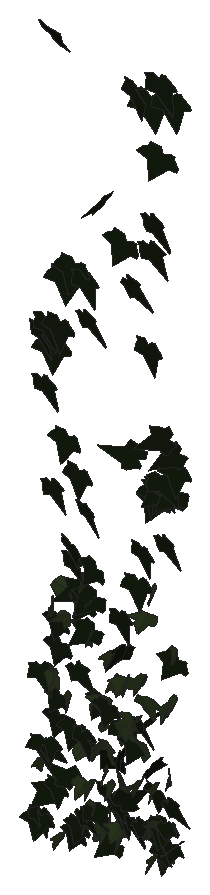
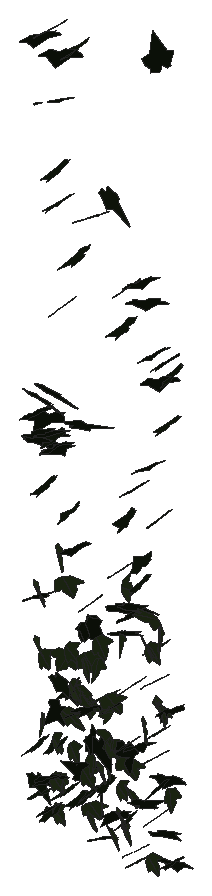
# SketchUp Ruby script. Lengths in inches.
U = 1.inch
M = Sketchup.active_model
def pt(a) = Geom::Point3d.new(a.map { |v| v * U })
def face(e, loops, mat)
  f = e.add_face(loops[0].map { |a| pt(a) })
  loops[1..].each { |l| e.add_face(l.map { |a| pt(a) }).erase! }
  f.material = f.back_material = mat if mat
  f
end
# faces: each face lists its corners as indices into pts; further lists are holes
def faces(e, pts, list, mat = nil) = list.each { |f| face(e, (f[0].is_a?(Array) ? f : [f]).map { |l| l.map { |i| pts[i] } }, mat) }
# xy, xz, yz: faces in a plane at the given z, y or x. An outline is a flat list of corners, or four numbers for a rectangle; further outlines are holes
def ring(l) = l.size == 4 ? [[l[0], l[1]], [l[2], l[1]], [l[2], l[3]], [l[0], l[3]]] : l.each_slice(2).to_a
def flat(e, list, mat, &to3) = list.each { |f| face(e, (f[0].is_a?(Array) ? f : [f]).map { |l| ring(l).map { |u, v| to3.(u, v) } }, mat) }
def xy(e, z, list, mat = nil) = flat(e, list, mat) { |x, y| [x, y, z] }
def xz(e, y, list, mat = nil) = flat(e, list, mat) { |x, z| [x, y, z] }
def yz(e, x, list, mat = nil) = flat(e, list, mat) { |y, z| [x, y, z] }
def lines(e, pts, list) = list.each { |a, b| e.add_line(pt(pts[a]), pt(pts[b])) }
# prism: a flat outline (further loops are holes) pulled along v
def prism(e, loops, v, mat = nil)
  f = face(e, loops, mat); d = Geom::Vector3d.new(v.map { |x| x * U })
  f.pushpull(f.normal.samedirection?(d) ? d.length : -d.length)
end
def box(e, o, s, mat = nil) = prism(e, [[o, [o[0] + s[0], o[1], o[2]], [o[0] + s[0], o[1] + s[1], o[2]], [o[0], o[1] + s[1], o[2]]]], [0, 0, s[2]], mat)
def at(x, y, z, deg = 0) = Geom::Transformation.translation(pt([x, y, z])) * Geom::Transformation.rotation(ORIGIN, Z_AXIS, deg.degrees)
def axes(o, x, y, z) = Geom::Transformation.new([*x, 0, *y, 0, *z, 0, *pt(o).to_a, 1])
def part(name) = M.definitions.add(name)
# library, detail: a bought-in or finely detailed component or shape, given as its bounding box
def library(name, o, s) = part(name).tap { |d| box(d.entities, o, s) }
def detail(e, o, s) = box(e.add_group.entities, o, s)
def put(e, d, t, mat = nil) = e.add_instance(d, t).tap { |i| i.material = mat if mat }
def group(e, t, mat = nil) = e.add_group.tap { |g| g.transformation = t; g.material = mat if mat }.entities
root = M.entities
M.materials.add("1026 AP 7946 SUNNY SIDE UP").color = [254, 231, 186]
M.materials.add("efeu1").color = [18, 25, 13]
M.materials.add("efeu2").color = [43, 57, 29]
c1 = part("ivyleaf_9")
p = [[1.54,2.16,1.25],[1.36,2.04,1.19],[-0.21,0.99,0.68],[-0.71,1.11,0.82],[-0.85,0.86,0.67],[-0.8,0.17,0.21],
  [-0.9,-0.01,0.1],[-0.67,-0.16,-0.02],[-0.08,-0.08,-0.05],[-0.03,-0.6,-0.4],[0.65,-0.88,-0.66],[0.83,-0.6,-0.49],
  [1.29,-0.42,-0.43],[1.8125,-0.07,-0.26],[1.21,0.44,0.15]]
faces(c1.entities,p,[[0,1,2,3,4,5,6,7,8,9,10,11,12,13,14]],"efeu1")
c2 = part("ivyleaf_10")
p = [[0,0.5,-0.03],[-0.0625,2.02,-0.43],[-0.19,2.01,-0.46],[-0.54,1.05,-0.29],[-0.52,0.625,-0.18],[-0.83,0.76,-0.28],
  [-1.16,0.64,-0.33],[-1.15,0.33,-0.24],[-0.77,-0.39,0.02],[-0.3,-0.51,0.16],[0.04,-0.48,0.23],[-0.02,2.01,-0.4375],
  [-0.06,2.01,-0.43],[0.04,-0.49,0.23],[0.67,-0.49,0.14],[1.38,0.36,-0.2],[1.375,0.51,-0.24],[0.81,0.65,-0.19],
  [0.62,0.59,-0.15],[0.6,1.09,-0.28],[0.5,1.23,-0.31]]
faces(c2.entities,p,[[0,1,2,3,4,5,6,7,8,9,10],[11,12,0,13,14,15,16,17,18,19,20]],"efeu2")
put(root,c1,axes([118.96,212.625,291.69],[0.00365,-0.3577,-0.01819],[0.01017,0.01567,-0.36835],[0.56289,0.00204,0.00677]),"1026 AP 7946 SUNNY SIDE UP")
put(root,c1,axes([119.125,212.41,291.59],[-0.41683,-0.22703,-0.10617],[0.19274,0.01023,-0.35238],[0.34043,-0.28377,0.06951]),"1026 AP 7946 SUNNY SIDE UP")
put(root,c1,axes([118.87,212.65,315.31],[0.20981,-0.41083,0.07483],[0.01065,-0.07657,-0.4451],[0.65657,0.13252,-0.01669]),"1026 AP 7946 SUNNY SIDE UP")
put(root,c1,axes([119.18,212.4,298.92],[-0.00879,-0.36906,-0.13016],[0.01023,0.12416,-0.3795],[0.61224,-0.00737,0.00447]),"1026 AP 7946 SUNNY SIDE UP")
put(root,c2,axes([119.4,212.16,294.67],[-0.0589,-0.36928,-0.07771],[0.03853,0.07115,-0.38157],[0.59074,-0.04146,0.01714]),"1026 AP 7946 SUNNY SIDE UP")
put(root,c1,axes([119.08,212.63,312.84],[0.20023,-0.41314,0.00123],[0.03723,0.0036,-0.44468],[0.64858,0.12734,0.02515]),"1026 AP 7946 SUNNY SIDE UP")
put(root,c1,axes([119.625,212.625,292.91],[-0.47533,-0.19178,0.08981],[-0.07174,-0.09117,-0.36558],[0.32412,-0.30143,0.05079]),"1026 AP 7946 SUNNY SIDE UP")
put(root,c1,axes([119.25,212.66,315.86],[0.07475,-0.4373,-0.03649],[-0.00062,0.03309,-0.45296],[0.68956,0.04743,0.00355]),"1026 AP 7946 SUNNY SIDE UP")
put(root,c1,axes([119.48,212.28,295.48],[-0.29395,-0.27444,-0.18053],[0.21651,0.11453,-0.33844],[0.46252,-0.22803,0.04369]),"1026 AP 7946 SUNNY SIDE UP")
put(root,c2,axes([119.64,212.49,298.83],[0.3553,-0.3055,-0.0603],[-0.00291,0.0689,-0.38899],[0.4886,0.22257,0.04153]),"1026 AP 7946 SUNNY SIDE UP")
put(root,c1,axes([119.57,212.32,295.24],[0.29152,-0.15965,-0.29131],[-0.19492,0.26508,-0.23712],[0.47059,0.20869,0.08224]),"1026 AP 7946 SUNNY SIDE UP")
put(root,c1,axes([119.67,212.66,314.85],[-0.26572,-0.39782,-0.07221],[0.05002,0.06018,-0.44489],[0.63259,-0.17186,0.00485]),"1026 AP 7946 SUNNY SIDE UP")
put(root,c1,axes([119.81,212.78,297.625],[-0.18055,-0.28615,0.22776],[-0.03288,-0.22799,-0.31422],[0.5692,-0.10393,0.05409]),"1026 AP 7946 SUNNY SIDE UP")
put(root,c1,axes([119.78,212.86,296.55],[-0.15027,-0.33014,0.15159],[0.00189,-0.15441,-0.35252],[0.56955,-0.08659,0.04116]),"1026 AP 7946 SUNNY SIDE UP")
put(root,c2,axes([119.92,212.2,302.37],[0.18565,-0.35673,-0.14226],[0.04747,0.1507,-0.37916],[0.59846,0.09871,0.0742]),"1026 AP 7946 SUNNY SIDE UP")
put(root,c2,axes([119.91,212.24,298.75],[0.51817,-0.19118,-0.02137],[-0.03149,0.00465,-0.39241],[0.30055,0.33009,-0.00427]),"1026 AP 7946 SUNNY SIDE UP")
put(root,c1,axes([119.68,212.4375,308.0625],[0.20165,-0.39278,-0.05654],[-0.01046,0.0532,-0.42522],[0.62304,0.12802,0.01116]),"1026 AP 7946 SUNNY SIDE UP")
put(root,c2,axes([120.03,212.25,298.87],[0.25373,-0.34513,-0.02903],[-0.04682,0.01498,-0.39184],[0.54224,0.16279,-0.02025]),"1026 AP 7946 SUNNY SIDE UP")
put(root,c1,axes([119.92,212.79,300.125],[-0.16934,-0.33464,0.16899],[-0.00213,-0.17235,-0.35997],[0.58733,-0.09711,0.04742]),"1026 AP 7946 SUNNY SIDE UP")
put(root,c1,axes([119.67,212.45,330.08],[0.64208,-0.18839,-0.15741],[0.24623,-0.02102,0.46093],[-0.28989,-0.43511,0.04286]),"1026 AP 7946 SUNNY SIDE UP")
put(root,c2,axes([120.14,212.61,301.58],[0.01087,-0.35287,0.17647],[0.00565,-0.17327,-0.36461],[0.61814,0.00779,0.00023]),"1026 AP 7946 SUNNY SIDE UP")
put(root,c1,axes([119.96,212.51,293.42],[-0.02179,-0.35642,0.10657],[-0.00696,-0.10538,-0.36808],[0.58442,-0.01455,-0.00041]),"1026 AP 7946 SUNNY SIDE UP")
put(root,c1,axes([119.97,212.66,315.95],[-0.09002,-0.43165,0.06713],[0.00279,-0.06842,-0.44884],[0.687,-0.05628,0.01062]),"1026 AP 7946 SUNNY SIDE UP")
put(root,c1,axes([120.07,212.45,301.55],[-0.14666,-0.32636,0.19998],[0.02445,-0.20487,-0.34505],[0.59808,-0.07165,0.06314]),"1026 AP 7946 SUNNY SIDE UP")
put(root,c2,axes([120.36,212.27,291.16],[-0.01751,-0.34657,0.10837],[-0.00014,-0.10721,-0.35783],[0.5704,-0.01067,0.00324]),"1026 AP 7946 SUNNY SIDE UP")
put(root,c1,axes([120.72,212.5,293.8125],[-0.08315,0.17554,0.32686],[-0.56814,-0.04091,-0.03908],[0.02719,-0.31806,0.18297]),"1026 AP 7946 SUNNY SIDE UP")
put(root,c2,axes([120.32,212.59,301.71],[0.47823,-0.22974,0.09619],[0.07621,-0.09191,-0.39072],[0.38321,0.30498,-0.04233]),"1026 AP 7946 SUNNY SIDE UP")
put(root,c1,axes([120.3,212.76,310.4],[-0.20744,-0.38508,0.1151],[0.01055,-0.122,-0.41758],[0.63136,-0.12448,0.04479]),"1026 AP 7946 SUNNY SIDE UP")
put(root,c2,axes([120,212.65,303.16],[-0.22612,-0.10451,-0.36375],[0.55616,-0.14264,-0.10592],[-0.1578,-0.35297,0.14792]),"1026 AP 7946 SUNNY SIDE UP")
put(root,c1,axes([120.34,212.74,318.45],[-0.33209,-0.38826,-0.07865],[0.14716,0.03256,-0.45007],[0.60386,-0.22145,0.06643]),"1026 AP 7946 SUNNY SIDE UP")
put(root,c2,axes([120.54,212.54,297.81],[0.2772,-0.33596,-0.06476],[0.01722,0.07413,-0.38784],[0.53661,0.17117,0.0459]),"1026 AP 7946 SUNNY SIDE UP")
put(root,c1,axes([120.71,212.86,291.18],[-0.17628,-0.29329,0.17103],[0.00192,-0.17703,-0.31917],[0.53122,-0.09669,0.05791]),"1026 AP 7946 SUNNY SIDE UP")
put(root,c1,axes([120.53,212.7,304.66],[0.24555,-0.37449,0.00065],[-0.01355,-0.00658,-0.41789],[0.5887,0.15605,-0.00989]),"1026 AP 7946 SUNNY SIDE UP")
put(root,c1,axes([120.8125,212.6,319.11],[-0.22944,-0.42315,0.05642],[0.00277,-0.06102,-0.46095],[0.67141,-0.14435,0.02119]),"1026 AP 7946 SUNNY SIDE UP")
put(root,c1,axes([120.89,212.86,291.62],[-0.16329,-0.3084,0.15046],[0.0019,-0.15479,-0.33278],[0.53774,-0.0931,0.04686]),"1026 AP 7946 SUNNY SIDE UP")
put(root,c1,axes([120.71,212.5,305.38],[0.07562,-0.32788,0.24609],[0.1049,-0.23278,-0.3417],[0.63094,0.078,0.02731]),"1026 AP 7946 SUNNY SIDE UP")
put(root,c1,axes([120.96,212.53,296.59],[-0.24985,-0.33792,0.05339],[-0.00361,-0.0582,-0.38433],[0.53801,-0.15732,0.02221]),"1026 AP 7946 SUNNY SIDE UP")
put(root,c1,axes([121.34,212.66,303.29],[-0.53404,-0.10777,0.17955],[-0.2243,-0.11946,-0.36191],[0.23245,-0.36286,0.06328]),"1026 AP 7946 SUNNY SIDE UP")
put(root,c2,axes([121.35,212.66,295.71],[-0.52216,-0.11186,0.14784],[-0.15149,-0.14669,-0.3468],[0.24363,-0.33096,0.10121]),"1026 AP 7946 SUNNY SIDE UP")
put(root,c1,axes([121.06,212.62,309.04],[-0.07517,-0.40613,0.09824],[0.00728,-0.09881,-0.42155],[0.65677,-0.04539,0.01592]),"1026 AP 7946 SUNNY SIDE UP")
put(root,c1,axes([121.08,212.44,299.54],[0.22093,-0.33802,-0.14286],[-0.01743,0.14253,-0.37383],[0.57309,0.13464,0.0437]),"1026 AP 7946 SUNNY SIDE UP")
put(root,c1,axes([121.38,212.72,302.77],[-0.22886,-0.31291,0.19734],[-0.09393,-0.18505,-0.35595],[0.57068,-0.15594,0.02055]),"1026 AP 7946 SUNNY SIDE UP")
put(root,c1,axes([121.63,212.41,296.27],[0.31136,0.07476,-0.32638],[-0.50778,-0.00524,-0.20895],[-0.06936,0.37393,0.0646]),"1026 AP 7946 SUNNY SIDE UP")
put(root,c2,axes([121.49,212.3,294.1],[0.49266,-0.22097,0.01489],[-0.01027,-0.03641,-0.39368],[0.34817,0.31159,-0.03268]),"1026 AP 7946 SUNNY SIDE UP")
put(root,c2,axes([121.51,212.59,304.08],[0.12813,-0.18833,0.35561],[0.19249,-0.324,-0.21312],[0.58914,0.14682,-0.00771]),"1026 AP 7946 SUNNY SIDE UP")
put(root,c1,axes([121.34,212.61,318.7],[0.11203,-0.44343,-0.00746],[0.00821,0.00563,-0.4626],[0.69724,0.07118,0.00665]),"1026 AP 7946 SUNNY SIDE UP")
put(root,c2,axes([121.71,212.37,292.3],[0.20343,-0.34177,-0.00696],[-0.01814,0.00078,-0.37631],[0.53714,0.12946,-0.01007]),"1026 AP 7946 SUNNY SIDE UP")
put(root,c1,axes([121.35,212.6,307.42],[0.28749,-0.36505,0.07187],[0.01856,-0.07431,-0.4204],[0.58471,0.18184,-0.02199]),"1026 AP 7946 SUNNY SIDE UP")
put(root,c1,axes([121.85,212.72,303.13],[-0.48471,-0.23503,0.09567],[-0.09875,-0.07279,-0.39928],[0.3857,-0.314,0.01799]),"1026 AP 7946 SUNNY SIDE UP")
put(root,c1,axes([121.48,212.42,296.48],[0.05337,-0.37671,0.01256],[-0.00681,-0.01478,-0.3897],[0.59273,0.03375,-0.00561]),"1026 AP 7946 SUNNY SIDE UP")
put(root,c1,axes([121.36,212.64,316.8],[0.36572,-0.37641,-0.04487],[-0.00436,0.04691,-0.45498],[0.59542,0.23154,0.02423]),"1026 AP 7946 SUNNY SIDE UP")
put(root,c1,axes([121.94,212.45,301.7],[-0.4765,-0.20531,0.15032],[-0.0886,-0.16899,-0.36359],[0.38711,-0.29139,0.10182]),"1026 AP 7946 SUNNY SIDE UP")
put(root,c1,axes([121.57,212.17,292.72],[0.30758,-0.28296,-0.12523],[-0.07539,0.11235,-0.35292],[0.47733,0.20008,0.02495]),"1026 AP 7946 SUNNY SIDE UP")
put(root,c2,axes([121.8,212.57,292.95],[0.35691,-0.28053,0.05375],[0.02069,-0.05834,-0.37112],[0.44866,0.22585,-0.02565]),"1026 AP 7946 SUNNY SIDE UP")
put(root,c2,axes([121.88,212.42,301.5],[0.15558,-0.36389,-0.13535],[0.04897,0.14058,-0.38215],[0.60526,0.08216,0.06571]),"1026 AP 7946 SUNNY SIDE UP")
put(root,c2,axes([121.91,212.41,294.18],[0.06672,-0.32436,0.18084],[0.08828,-0.17082,-0.33663],[0.57456,0.06391,0.03072]),"1026 AP 7946 SUNNY SIDE UP")
put(root,c1,axes([121.98,212.57,304.65],[-0.20491,-0.28342,0.26401],[-0.06932,-0.25948,-0.31826],[0.59851,-0.12709,0.05352]),"1026 AP 7946 SUNNY SIDE UP")
put(root,c1,axes([122.47,212.55,322.78],[-0.38972,0.36724,-0.13204],[0.0869,-0.11968,-0.45665],[-0.60651,-0.25313,0.01942]),"1026 AP 7946 SUNNY SIDE UP")
put(root,c1,axes([122.14,212.8,298.13],[-0.17878,-0.29789,0.206],[-0.06369,-0.19954,-0.32836],[0.56204,-0.11737,0.02832]),"1026 AP 7946 SUNNY SIDE UP")
put(root,c2,axes([122.36,212.5,291.95],[0.31334,-0.25713,-0.15178],[-0.1561,0.10749,-0.33429],[0.43785,0.22234,-0.01056]),"1026 AP 7946 SUNNY SIDE UP")
put(root,c1,axes([122.01,212.51,292.94],[0.01394,-0.29872,-0.22071],[0.06352,0.21211,-0.30413],[0.57296,-0.01624,0.03909]),"1026 AP 7946 SUNNY SIDE UP")
put(root,c2,axes([122.39,212.56,298.375],[-0.31974,-0.24892,0.21264],[-0.08187,-0.21705,-0.32158],[0.50326,-0.19346,0.08278]),"1026 AP 7946 SUNNY SIDE UP")
put(root,c2,axes([122.3125,212.59,296.14],[0.05591,-0.33799,0.16614],[0.00806,-0.16347,-0.3509],[0.59011,0.03426,-0.01095]),"1026 AP 7946 SUNNY SIDE UP")
put(root,c2,axes([122.73,212.16,297.47],[0.11298,-0.11873,0.38046],[-0.17566,0.35406,0.14148],[-0.58519,-0.1292,0.03099]),"1026 AP 7946 SUNNY SIDE UP")
put(root,c2,axes([122.84,212.1875,295.09],[0.16419,-0.32606,-0.15629],[-0.06509,0.14409,-0.35184],[0.56049,0.11225,0.00492]),"1026 AP 7946 SUNNY SIDE UP")
put(root,c2,axes([122.63,212.39,296.34],[-0.43482,0.206,-0.17281],[0.19632,-0.11485,-0.35554],[-0.37002,-0.303,0.01443]),"1026 AP 7946 SUNNY SIDE UP")
put(root,c1,axes([122.52,212.52,294.11],[0.22696,-0.33999,0.06624],[0.02064,-0.06633,-0.38064],[0.54426,0.14429,-0.01318]),"1026 AP 7946 SUNNY SIDE UP")
put(root,c1,axes([122.95,212.68,291.47],[-0.39015,-0.19776,0.1727],[-0.08869,-0.18678,-0.31201],[0.39906,-0.23486,0.0995]),"1026 AP 7946 SUNNY SIDE UP")
put(root,c1,axes([123.11,212.33,295.91],[0.31095,0.0823,-0.34459],[-0.48386,-0.13234,-0.22143],[-0.24502,0.36578,-0.00005]),"1026 AP 7946 SUNNY SIDE UP")
put(root,c1,axes([122.8,212.48,298.27],[-0.1696,-0.33259,0.16115],[0.03445,-0.17047,-0.35454],[0.57816,-0.0874,0.0684]),"1026 AP 7946 SUNNY SIDE UP")
put(root,c2,axes([123,212.5,300.88],[-0.1028,-0.38024,0.08989],[-0.00154,-0.0905,-0.39773],[0.61419,-0.06387,0.01405]),"1026 AP 7946 SUNNY SIDE UP")
put(root,c2,axes([123.17,212.2,294.54],[0.27275,-0.33466,-0.03014],[-0.04465,0.01606,-0.3878],[0.52609,0.17487,-0.01729]),"1026 AP 7946 SUNNY SIDE UP")
put(root,c1,axes([122.93,212.39,293.12],[-0.00012,-0.06442,-0.40097],[0.54658,-0.18331,0.03015],[-0.29215,-0.34293,0.05656]),"1026 AP 7946 SUNNY SIDE UP")
put(root,c2,axes([123.21,212.32,299.7],[-0.01279,-0.36256,-0.14947],[0.13986,0.13756,-0.36362],[0.59667,-0.04002,0.08203]),"1026 AP 7946 SUNNY SIDE UP")
put(root,c2,axes([123.39,212.47,295.07],[-0.37869,0.2657,0.07516],[-0.12688,0.02256,-0.36654],[-0.4136,-0.25019,0.04363]),"1026 AP 7946 SUNNY SIDE UP")
put(root,c2,axes([123.57,212.29,292.65],[-0.36013,-0.21507,0.18486],[-0.03989,-0.21632,-0.29969],[0.43985,-0.19571,0.12418]),"1026 AP 7946 SUNNY SIDE UP")
put(root,c1,axes([123.27,212.66,302.78],[0.1049,-0.38824,-0.00692],[-0.00737,0.00377,-0.40578],[0.61047,0.06676,-0.00371]),"1026 AP 7946 SUNNY SIDE UP")
put(root,c1,axes([123.57,212.1875,295.75],[-0.02853,0.02099,0.41075],[0.21083,0.37614,-0.01191],[-0.59115,0.13313,-0.02407]),"1026 AP 7946 SUNNY SIDE UP")
put(root,c2,axes([123.59,212.64,294.36],[-0.0553,-0.33434,0.15356],[0.02271,-0.1528,-0.34605],[0.57638,-0.02605,0.02837]),"1026 AP 7946 SUNNY SIDE UP")
put(root,c1,axes([123.36,212.47,293.52],[0.03086,-0.35536,0.10153],[0.00697,-0.10048,-0.36723],[0.58067,0.02009,-0.00099]),"1026 AP 7946 SUNNY SIDE UP")
put(root,c2,axes([123.54,212.42,292.17],[0.28201,-0.30074,0.14689],[0.07951,-0.13742,-0.36061],[0.51843,0.18467,-0.0246]),"1026 AP 7946 SUNNY SIDE UP")
put(root,c1,axes([123.74,212.35,301.42],[-0.08698,0.20204,-0.35405],[0.14345,-0.33254,-0.21775],[-0.61183,-0.10669,-0.00072]),"1026 AP 7946 SUNNY SIDE UP")
put(root,c2,axes([123.75,212.41,299.85],[-0.30718,-0.30203,0.16147],[-0.03944,-0.16939,-0.36547],[0.53486,-0.18595,0.06579]),"1026 AP 7946 SUNNY SIDE UP")
put(root,c2,axes([123.67,212.62,299.67],[0.14416,-0.37457,-0.03441],[0.00802,0.03343,-0.39686],[0.59097,0.09092,0.01378]),"1026 AP 7946 SUNNY SIDE UP")
put(root,c1,axes([123.62,212.58,321.24],[-0.32978,-0.36402,0.18428],[0.00209,-0.20422,-0.42286],[0.6392,-0.18714,0.09645]),"1026 AP 7946 SUNNY SIDE UP")
put(root,c1,axes([123.77,212.34,301.45],[-0.15836,0.16723,-0.36301],[0.22679,-0.32321,-0.20185],[-0.57128,-0.17467,0.0205]),"1026 AP 7946 SUNNY SIDE UP")
put(root,c2,axes([123.83,212.19,297.61],[-0.5731,0.11691,0.04706],[-0.11371,-0.08327,-0.38093],[-0.16085,-0.35768,0.10164]),"1026 AP 7946 SUNNY SIDE UP")
put(root,c1,axes([123.55,212.55,297.53],[-0.0751,-0.35903,-0.13793],[0.11741,0.12157,-0.36817],[0.58983,-0.06991,0.05572]),"1026 AP 7946 SUNNY SIDE UP")
put(root,c1,axes([124.34,212.44,310.9],[-0.34403,0.1329,0.34342],[-0.56288,-0.09406,-0.20442],[0.01867,-0.38684,0.16503]),"1026 AP 7946 SUNNY SIDE UP")
put(root,c1,axes([123.64,212.48,293.13],[0.06441,-0.32697,0.169],[0.04441,-0.16363,-0.34036],[0.57482,0.04928,0.00736]),"1026 AP 7946 SUNNY SIDE UP")
put(root,c2,axes([124.15,212.23,298.07],[0.37027,-0.2108,-0.25052],[-0.31215,0.14014,-0.32397],[0.39649,0.30719,-0.0211]),"1026 AP 7946 SUNNY SIDE UP")
put(root,c1,axes([123.91,212.04,294.05],[-0.08074,0.0281,0.4107],[0.5812,0.15578,0.03866],[-0.23833,0.37037,-0.04486]),"1026 AP 7946 SUNNY SIDE UP")
put(root,c1,axes([123.89,212.52,319.37],[0.42863,-0.33434,-0.13808],[-0.06895,0.13366,-0.44084],[0.56106,0.27185,0.05131]),"1026 AP 7946 SUNNY SIDE UP")
put(root,c1,axes([124,212.58,292.96],[0.24318,-0.33295,0.018],[-0.00793,-0.02367,-0.37804],[0.52435,0.15406,-0.01406]),"1026 AP 7946 SUNNY SIDE UP")
put(root,c2,axes([124.7,212.46,296.8],[0.23647,-0.02598,-0.34941],[-0.44918,0.19139,-0.14454],[0.28996,0.31768,0.06105]),"1026 AP 7946 SUNNY SIDE UP")
put(root,c1,axes([124.32,212.49,296.95],[-0.25178,-0.32217,0.12604],[-0.01988,-0.13132,-0.36855],[0.54255,-0.15433,0.04499]),"1026 AP 7946 SUNNY SIDE UP")
put(root,c2,axes([124.47,212.4,298.16],[0.12468,-0.35589,0.11623],[0.03189,-0.11313,-0.37626],[0.58715,0.08171,-0.00424]),"1026 AP 7946 SUNNY SIDE UP")
put(root,c2,axes([124.47,212.67,300.09],[-0.00918,-0.32644,0.21054],[0.06757,-0.20552,-0.33509],[0.60337,0.01805,0.04073]),"1026 AP 7946 SUNNY SIDE UP")
put(root,c2,axes([124.54,212.38,295.17],[0.01917,-0.36944,0.0552],[-0.00387,-0.05579,-0.38111],[0.58746,0.01169,-0.00431]),"1026 AP 7946 SUNNY SIDE UP")
put(root,c1,axes([124.43,212.43,304.9375],[-0.1058,-0.40652,-0.01353],[0.01025,0.00989,-0.42441],[0.63936,-0.06743,0.00457]),"1026 AP 7946 SUNNY SIDE UP")
put(root,c1,axes([124.37,212.43,329.04],[0.03149,-0.45298,0.15911],[0.037,-0.15603,-0.46775],[0.75294,0.02661,0.01633]),"1026 AP 7946 SUNNY SIDE UP")
put(root,c2,axes([124.77,212.59,303.26],[-0.39023,-0.2683,0.1618],[-0.05264,-0.1786,-0.3663],[0.48723,-0.23419,0.09002]),"1026 AP 7946 SUNNY SIDE UP")
put(root,c1,axes([124.5,212.38,298.11],[0.35611,-0.30681,-0.04738],[-0.07917,0.01767,-0.39155],[0.48095,0.23008,-0.02937]),"1026 AP 7946 SUNNY SIDE UP")
put(root,c1,axes([124.6,212.29,293.19],[0.31748,-0.27689,-0.1503],[-0.03721,0.1578,-0.34508],[0.48957,0.19156,0.07124]),"1026 AP 7946 SUNNY SIDE UP")
put(root,c1,axes([124.61,212.48,306.53],[0.11579,-0.39089,0.12008],[0.03025,-0.11724,-0.41045],[0.64167,0.07606,-0.00232]),"1026 AP 7946 SUNNY SIDE UP")
put(root,c1,axes([125.18,212.59,298.39],[-0.3372,0.30847,-0.10037],[0.03193,-0.10591,-0.38519],[-0.5085,-0.21121,0.04237]),"1026 AP 7946 SUNNY SIDE UP")
put(root,c2,axes([125.02,212.24,299.4],[-0.59579,0.07828,-0.09218],[0.12719,-0.05127,-0.39744],[-0.1377,-0.38604,0.0317]),"1026 AP 7946 SUNNY SIDE UP")
put(root,c2,axes([125.14,212.59,304.61],[0.19845,-0.37347,-0.08973],[-0.03186,0.08284,-0.40557],[0.60142,0.12762,0.00812]),"1026 AP 7946 SUNNY SIDE UP")
put(root,c1,axes([124.86,212.62,316.55],[0.04943,-0.43798,0.0655],[-0.00029,-0.06625,-0.45272],[0.69647,0.03106,-0.00484]),"1026 AP 7946 SUNNY SIDE UP")
put(root,c1,axes([125.05,212.57,328.78],[-0.28016,-0.41257,-0.17385],[0.12203,0.14769,-0.46194],[0.68878,-0.19397,0.01112]),"1026 AP 7946 SUNNY SIDE UP")
put(root,c2,axes([125.27,212.05,293.31],[0.12492,-0.31163,-0.17412],[0.05631,0.17762,-0.32239],[0.55326,0.05229,0.07213]),"1026 AP 7946 SUNNY SIDE UP")
put(root,c2,axes([125.41,212.44,293.39],[-0.01528,-0.3334,0.16706],[-0.00599,-0.16402,-0.34457],[0.58424,-0.0104,0.00084]),"1026 AP 7946 SUNNY SIDE UP")
put(root,c1,axes([125.03,212.51,321.5],[0.21215,-0.43348,-0.0599],[0.03734,0.06546,-0.46533],[0.68619,0.13046,0.04384]),"1026 AP 7946 SUNNY SIDE UP")
put(root,c2,axes([125.43,212.33,291.8],[0.08577,-0.33417,0.14826],[0.01473,-0.1461,-0.34941],[0.57311,0.05377,-0.01321]),"1026 AP 7946 SUNNY SIDE UP")
put(root,c1,axes([125.33,212.62,309.56],[-0.21417,-0.39223,0.05868],[-0.00922,-0.06059,-0.42784],[0.62365,-0.13559,0.01383]),"1026 AP 7946 SUNNY SIDE UP")
put(root,c2,axes([125.4,212.42,295.24],[0.13919,-0.31867,0.18401],[0.0962,-0.17014,-0.3415],[0.56772,0.10696,0.01275]),"1026 AP 7946 SUNNY SIDE UP")
put(root,c1,axes([125.86,212.66,312.28],[-0.6519,0.08352,0.08539],[-0.1442,-0.04188,-0.43181],[-0.11509,-0.42062,0.05736]),"1026 AP 7946 SUNNY SIDE UP")
put(root,c1,axes([125.49,212.52,309.38],[-0.32545,-0.35402,0.08546],[-0.04754,-0.08068,-0.42268],[0.57049,-0.20868,0.01353]),"1026 AP 7946 SUNNY SIDE UP")
put(root,c1,axes([125.21,212.38,322.96],[0.31232,-0.4149,-0.03861],[-0.0084,0.03638,-0.47354],[0.65467,0.1984,0.01235]),"1026 AP 7946 SUNNY SIDE UP")
put(root,c1,axes([125.36,212.53,294.97],[-0.02115,-0.32467,0.19029],[0.07934,-0.18655,-0.3318],[0.58342,0.0136,0.05202]),"1026 AP 7946 SUNNY SIDE UP")
put(root,c1,axes([125.66,211.84,296.51],[-0.11391,0.09763,-0.38477],[-0.26428,0.33476,0.12551],[0.54741,0.18193,-0.01948]),"1026 AP 7946 SUNNY SIDE UP")
put(root,c1,axes([125.41,212.8,291.78],[-0.0146,-0.28695,0.21647],[0.09192,-0.21019,-0.29201],[0.55317,0.02735,0.05424]),"1026 AP 7946 SUNNY SIDE UP")
put(root,c1,axes([125.31,212.58,309.99],[0.23086,-0.39047,0.05502],[0.13063,-0.02741,-0.42425],[0.60626,0.15459,0.07046]),"1026 AP 7946 SUNNY SIDE UP")
put(root,c1,axes([125.67,212.57,326.19],[-0.40323,-0.37318,0.12802],[0.04807,-0.16919,-0.45174],[0.61766,-0.23045,0.11873]),"1026 AP 7946 SUNNY SIDE UP")
put(root,c1,axes([125.59,212.75,291.97],[-0.08274,-0.34381,0.09654],[-0.01765,-0.09505,-0.35886],[0.56087,-0.05371,0.00295]),"1026 AP 7946 SUNNY SIDE UP")
put(root,c1,axes([125.67,212.55,293.43],[-0.26916,-0.3279,-0.03309],[0.0383,0.0214,-0.38074],[0.51636,-0.17251,0.011]),"1026 AP 7946 SUNNY SIDE UP")
put(root,c1,axes([125.87,212.44,309.96],[-0.44917,-0.25979,0.17113],[-0.1078,-0.16927,-0.39169],[0.47402,-0.28467,0.07309]),"1026 AP 7946 SUNNY SIDE UP")
put(root,c1,axes([125.49,212.5625,329.79],[0.09723,-0.47711,-0.02896],[0.06247,0.03066,-0.49343],[0.74866,0.0594,0.04493]),"1026 AP 7946 SUNNY SIDE UP")
put(root,c1,axes([125.73,212.78,293.35],[-0.18861,-0.33841,0.07647],[-0.00058,-0.08045,-0.36938],[0.54543,-0.11711,0.02605]),"1026 AP 7946 SUNNY SIDE UP")
put(root,c2,axes([125.92,212.62,299.26],[-0.00607,-0.34237,0.1689],[0.08296,-0.16478,-0.35004],[0.59243,0.01957,0.05075]),"1026 AP 7946 SUNNY SIDE UP")
put(root,c1,axes([126.24,212.73,309.7],[-0.60323,-0.16582,0.03562],[-0.01582,-0.06545,-0.42707],[0.26618,-0.37968,0.05535]),"1026 AP 7946 SUNNY SIDE UP")
put(root,c1,axes([126.42,212.66,311.76],[-0.6673,0.03195,-0.01391],[0.01239,-0.07489,-0.43219],[-0.05323,-0.41795,0.07384]),"1026 AP 7946 SUNNY SIDE UP")
put(root,c1,axes([125.84,212.39,307.47],[0.29901,-0.37034,-0.03807],[-0.01467,0.03438,-0.42861],[0.58471,0.19025,0.00871]),"1026 AP 7946 SUNNY SIDE UP")
put(root,c2,axes([126.2,212.32,296.02],[0.16696,-0.29738,-0.21768],[0.01863,0.22106,-0.31563],[0.57178,0.07963,0.07384]),"1026 AP 7946 SUNNY SIDE UP")
put(root,c1,axes([125.99,212.17,310.69],[-0.06948,-0.34987,-0.27073],[0.05105,0.25878,-0.36179],[0.68427,-0.05483,-0.0005]),"1026 AP 7946 SUNNY SIDE UP")
put(root,c1,axes([126.09,212.69,292.51],[-0.14697,-0.31571,0.16234],[0.07277,-0.17435,-0.32886],[0.55131,-0.06115,0.08668]),"1026 AP 7946 SUNNY SIDE UP")
put(root,c1,axes([126.42,212.6875,309.89],[-0.41861,-0.2773,0.17272],[-0.14454,-0.14556,-0.39553],[0.48993,-0.27987,0.03089]),"1026 AP 7946 SUNNY SIDE UP")
put(root,c2,axes([126.3,212.56,299.7],[0.30823,-0.32698,0.05505],[0.01542,-0.05849,-0.39247],[0.52122,0.1951,-0.02094]),"1026 AP 7946 SUNNY SIDE UP")
put(root,c1,axes([126.18,212.53,329.17],[-0.16015,-0.45797,-0.10276],[0.06406,0.09038,-0.48237],[0.73335,-0.1079,0.01969]),"1026 AP 7946 SUNNY SIDE UP")
put(root,c1,axes([126.27,212.77,310.97],[-0.14536,-0.41134,0.03056],[0.00691,-0.03377,-0.43436],[0.64871,-0.09181,0.01147]),"1026 AP 7946 SUNNY SIDE UP")
put(root,c1,axes([126.69,212.07,292.84],[-0.16387,0.34267,-0.04897],[-0.01044,-0.05364,-0.36862],[-0.54431,-0.10213,0.02181]),"1026 AP 7946 SUNNY SIDE UP")
put(root,c2,axes([126.46,212.32,302.2],[0.36786,-0.32296,0.0416],[0.01354,-0.04582,-0.41059],[0.51196,0.23327,-0.01903]),"1026 AP 7946 SUNNY SIDE UP")
put(root,c1,axes([126.57,212.44,301.81],[-0.33345,-0.29026,0.16278],[-0.04349,-0.17339,-0.36361],[0.51907,-0.20099,0.0741]),"1026 AP 7946 SUNNY SIDE UP")
put(root,c1,axes([126.3125,212.24,294.78],[0.33849,-0.27696,-0.14314],[-0.06815,0.13871,-0.35725],[0.48132,0.21441,0.05008]),"1026 AP 7946 SUNNY SIDE UP")
